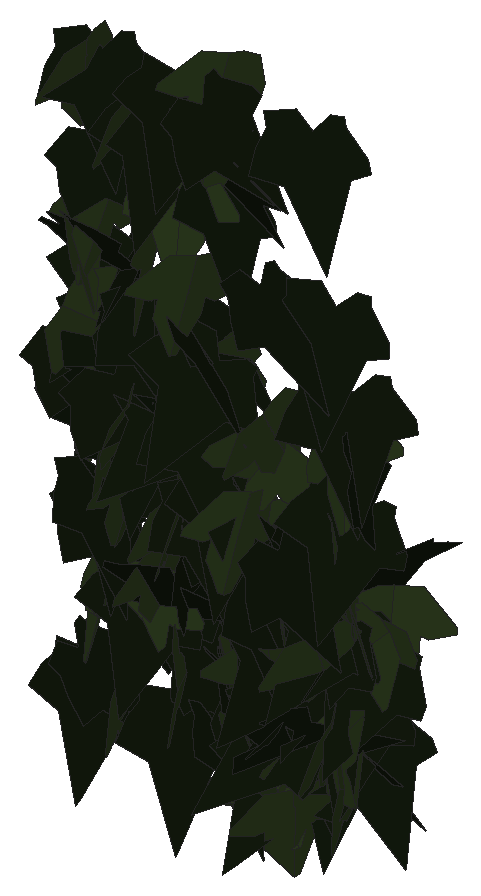
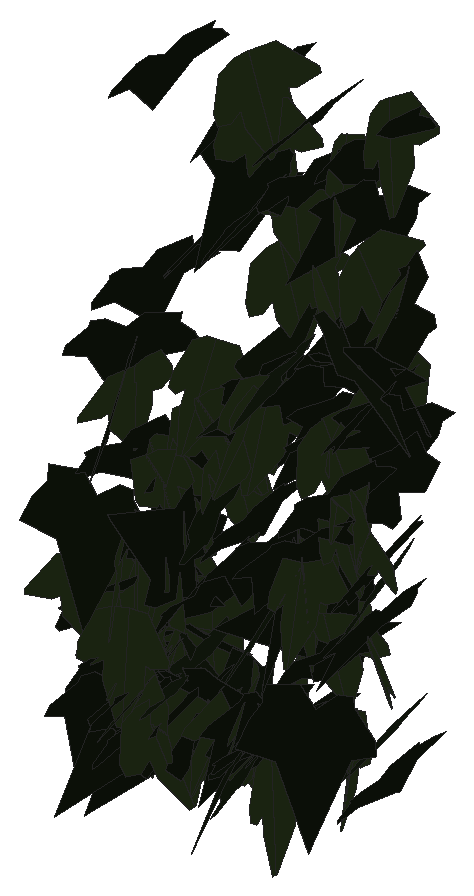
# SketchUp Ruby script. Lengths in inches.
U = 1.inch
M = Sketchup.active_model
def pt(a) = Geom::Point3d.new(a.map { |v| v * U })
def face(e, loops, mat)
  f = e.add_face(loops[0].map { |a| pt(a) })
  loops[1..].each { |l| e.add_face(l.map { |a| pt(a) }).erase! }
  f.material = f.back_material = mat if mat
  f
end
# faces: each face lists its corners as indices into pts; further lists are holes
def faces(e, pts, list, mat = nil) = list.each { |f| face(e, (f[0].is_a?(Array) ? f : [f]).map { |l| l.map { |i| pts[i] } }, mat) }
# xy, xz, yz: faces in a plane at the given z, y or x. An outline is a flat list of corners, or four numbers for a rectangle; further outlines are holes
def ring(l) = l.size == 4 ? [[l[0], l[1]], [l[2], l[1]], [l[2], l[3]], [l[0], l[3]]] : l.each_slice(2).to_a
def flat(e, list, mat, &to3) = list.each { |f| face(e, (f[0].is_a?(Array) ? f : [f]).map { |l| ring(l).map { |u, v| to3.(u, v) } }, mat) }
def xy(e, z, list, mat = nil) = flat(e, list, mat) { |x, y| [x, y, z] }
def xz(e, y, list, mat = nil) = flat(e, list, mat) { |x, z| [x, y, z] }
def yz(e, x, list, mat = nil) = flat(e, list, mat) { |y, z| [x, y, z] }
def lines(e, pts, list) = list.each { |a, b| e.add_line(pt(pts[a]), pt(pts[b])) }
# prism: a flat outline (further loops are holes) pulled along v
def prism(e, loops, v, mat = nil)
  f = face(e, loops, mat); d = Geom::Vector3d.new(v.map { |x| x * U })
  f.pushpull(f.normal.samedirection?(d) ? d.length : -d.length)
end
def box(e, o, s, mat = nil) = prism(e, [[o, [o[0] + s[0], o[1], o[2]], [o[0] + s[0], o[1] + s[1], o[2]], [o[0], o[1] + s[1], o[2]]]], [0, 0, s[2]], mat)
def at(x, y, z, deg = 0) = Geom::Transformation.translation(pt([x, y, z])) * Geom::Transformation.rotation(ORIGIN, Z_AXIS, deg.degrees)
def axes(o, x, y, z) = Geom::Transformation.new([*x, 0, *y, 0, *z, 0, *pt(o).to_a, 1])
def part(name) = M.definitions.add(name)
# library, detail: a bought-in or finely detailed component or shape, given as its bounding box
def library(name, o, s) = part(name).tap { |d| box(d.entities, o, s) }
def detail(e, o, s) = box(e.add_group.entities, o, s)
def put(e, d, t, mat = nil) = e.add_instance(d, t).tap { |i| i.material = mat if mat }
def group(e, t, mat = nil) = e.add_group.tap { |g| g.transformation = t; g.material = mat if mat }.entities
root = M.entities
M.materials.add("efeu1").color = [18, 25, 13]
M.materials.add("efeu2").color = [43, 57, 29]
c1 = part("ivyleaf_9")
p = [[1.54,2.16,1.25],[1.36,2.04,1.19],[-0.21,0.99,0.68],[-0.71,1.11,0.82],[-0.85,0.86,0.67],[-0.8,0.17,0.21],
  [-0.9,-0.01,0.1],[-0.67,-0.16,-0.02],[-0.08,-0.08,-0.05],[-0.03,-0.6,-0.4],[0.65,-0.88,-0.66],[0.83,-0.6,-0.49],
  [1.29,-0.42,-0.43],[1.8125,-0.07,-0.26],[1.21,0.44,0.15]]
faces(c1.entities,p,[[0,1,2,3,4,5,6,7,8,9,10,11,12,13,14]],"efeu1")
c2 = part("ivyleaf_10")
p = [[0,0.5,-0.03],[-0.0625,2.02,-0.43],[-0.19,2.01,-0.46],[-0.54,1.05,-0.29],[-0.52,0.625,-0.18],[-0.83,0.76,-0.28],
  [-1.16,0.64,-0.33],[-1.15,0.33,-0.24],[-0.77,-0.39,0.02],[-0.3,-0.51,0.16],[0.04,-0.48,0.23],[-0.02,2.01,-0.4375],
  [-0.06,2.01,-0.43],[0.04,-0.49,0.23],[0.67,-0.49,0.14],[1.38,0.36,-0.2],[1.375,0.51,-0.24],[0.81,0.65,-0.19],
  [0.62,0.59,-0.15],[0.6,1.09,-0.28],[0.5,1.23,-0.31]]
faces(c2.entities,p,[[0,1,2,3,4,5,6,7,8,9,10],[11,12,0,13,14,15,16,17,18,19,20]],"efeu2")
put(root,c1,axes([30.55,222.95,235.93],[0.19386,-0.41787,-0.19443],[-0.01892,0.20353,-0.45631],[0.4605,0.18427,0.0631]))
put(root,c2,axes([30.73,222.43,239.54],[-0.161,0.47233,-0.03139],[0.01068,-0.02953,-0.49901],[-0.47325,-0.16135,-0.00058]))
put(root,c2,axes([30.82,222.4,241.56],[-0.01451,-0.49272,-0.08377],[0.02037,0.08315,-0.49262],[0.49937,-0.01771,0.01766]))
put(root,c1,axes([30.64,222.81,233.83],[-0.031,-0.48215,0.12872],[0.01205,-0.12966,-0.48275],[0.49889,-0.02683,0.01966]))
put(root,c2,axes([30.57,223.07,236.89],[0.34889,-0.11485,0.33924],[0.31911,-0.11535,-0.36724],[0.16261,0.47276,-0.00719]))
put(root,c1,axes([31.01,222.9,238.78],[-0.45891,-0.19762,-0.01859],[0.01587,0.01014,-0.49965],[0.19786,-0.45918,-0.00303]))
put(root,c1,axes([30.65,222.49,238.12],[0.11578,-0.27785,-0.39924],[0.07613,0.41569,-0.26722],[0.48042,0.00109,0.13856]))
put(root,c1,axes([30.69,222.55,234.3],[0.33786,-0.2932,-0.22335],[-0.07021,0.24625,-0.42946],[0.36183,0.32155,0.12523]))
put(root,c1,axes([30.61,222.39,239.41],[0.48865,-0.03264,0.10078],[0.10352,0.04619,-0.48698],[0.02248,0.49679,0.0519]))
put(root,c1,axes([31.18,222.78,239.02],[-0.34279,0.364,0.00184],[-0.00557,-0.00272,-0.49996],[-0.36396,-0.34278,0.00592]))
put(root,c2,axes([30.81,222.3,238.54],[-0.08236,-0.30647,-0.38639],[0.21642,0.32954,-0.30751],[0.44315,-0.2179,0.07837]))
put(root,c1,axes([30.73,222.92,235.98],[0.09408,-0.44344,0.21097],[0.04085,-0.20699,-0.45331],[0.48937,0.10253,-0.00272]))
put(root,c2,axes([30.97,222.63,239.85],[-0.08362,-0.45117,0.19862],[0.05349,-0.20858,-0.45126],[0.49005,-0.05422,0.08315]))
put(root,c1,axes([31.04,223.44,234.74],[0.279,0.35016,-0.22258],[-0.13361,-0.17811,-0.44769],[-0.39282,0.30929,-0.00582]))
put(root,c1,axes([30.77,222.76,238.31],[0.17898,-0.45059,-0.1222],[-0.01558,0.12504,-0.48386],[0.46661,0.17701,0.03072]))
put(root,c2,axes([30.92,222.64,235.36],[0.36046,-0.31356,0.14749],[0.09884,-0.11095,-0.47741],[0.33212,0.37333,-0.018]))
put(root,c1,axes([30.86,222.68,241.45],[-0.01708,-0.48793,-0.10783],[0.00054,0.10788,-0.48822],[0.49971,-0.01679,-0.00316]))
put(root,c1,axes([30.83,222.6,236.33],[0.14816,-0.47731,-0.01509],[-0.00189,0.01521,-0.49977],[0.47754,0.14815,0.0027]))
put(root,c2,axes([31.15,222.34,237.14],[0.18383,-0.33982,-0.31738],[-0.04232,0.32764,-0.37531],[0.46305,0.16485,0.0917]))
put(root,c2,axes([31.19,222.97,237.81],[-0.168,-0.44111,0.16491],[0.01098,-0.17872,-0.46684],[0.4708,-0.15323,0.06974]))
put(root,c2,axes([31.18,222.54,234.0625],[0.20112,-0.37951,-0.25598],[0.00848,0.28264,-0.41236],[0.45769,0.16152,0.12013]))
put(root,c1,axes([30.98,222.48,240.6],[0.10051,-0.28357,-0.39935],[0.0266,0.41023,-0.28461],[0.48907,0.03597,0.09755]))
put(root,c1,axes([30.8125,222.39,237.12],[0.07192,-0.02937,0.49393],[0.47234,-0.14459,-0.07737],[0.14738,0.47774,0.00695]))
put(root,c1,axes([31.13,223.06,237.22],[-0.09608,-0.49043,-0.01568],[-0.00654,0.01726,-0.49966],[0.49064,-0.09581,-0.00973]))
put(root,c2,axes([31.29,222.5625,241.02],[0.04981,-0.44926,-0.21373],[0.00318,0.21508,-0.45136],[0.4975,0.0436,0.02428]))
put(root,c2,axes([31.35,222.48,237.45],[0.024,-0.39949,-0.29972],[-0.01831,0.29916,-0.40021],[0.49909,0.03019,-0.00026]))
put(root,c2,axes([31.4,222.55,236.73],[0.02853,-0.49666,0.0502],[-0.00165,-0.05037,-0.49745],[0.49918,0.02822,-0.00451]))
put(root,c1,axes([31.38,222.87,235.125],[-0.14875,-0.47153,0.07437],[0.01814,-0.08343,-0.49266],[0.47702,-0.14387,0.04193]))
put(root,c2,axes([31.46,222.64,235.29],[0.47155,0.16207,-0.03714],[-0.03748,-0.00522,-0.49857],[-0.16199,0.47298,0.00722]))
put(root,c2,axes([31.53,223.02,236.11],[-0.06155,-0.46338,-0.17744],[0.05462,0.17139,-0.46652],[0.49318,-0.07682,0.02952]))
put(root,c1,axes([31.3,222.375,237.85],[0.04457,-0.30022,-0.39734],[0.10509,0.39562,-0.28713],[0.4868,-0.05792,0.09836]))
put(root,c1,axes([31.4,222.84,238.54],[0.02355,-0.45825,-0.19863],[0.01148,0.1993,-0.45842],[0.49931,0.01703,0.01991]))
put(root,c2,axes([31.63,223.375,233.73],[0.01446,-0.48813,-0.10733],[0.00744,0.10758,-0.48823],[0.49974,0.01252,0.01038]))
put(root,c1,axes([31.43,223.23,236.5625],[0.03208,-0.45675,-0.20087],[0.05566,0.2033,-0.4534],[0.49586,0.00673,0.06388]))
put(root,c2,axes([31.71,222.61,235.76],[-0.02973,-0.49429,-0.06923],[0.01444,0.06848,-0.49508],[0.49891,-0.03144,0.0102]))
put(root,c1,axes([31.61,222.86,240.84],[-0.18609,-0.46401,0.00784],[0.00313,-0.0097,-0.4999],[0.46407,-0.186,0.00651]))
put(root,c2,axes([31.59,222.62,239.53],[0.19992,-0.39705,0.22888],[0.14752,-0.18067,-0.44226],[0.4339,0.24436,0.04491]))
put(root,c2,axes([31.8,222.7,236.28],[0.21002,-0.40487,-0.20487],[-0.06846,0.19489,-0.45533],[0.44856,0.21931,0.02643]))
put(root,c1,axes([31.92,222.71,235.84],[0.06542,0.0152,-0.49547],[-0.42118,0.26524,-0.04747],[0.2614,0.42357,0.04751]))
put(root,c1,axes([31.41,222.43,235.37],[0.39266,-0.0311,0.30798],[0.30948,0.05005,-0.38951],[-0.0066,0.49652,0.05855]))
put(root,c1,axes([31.625,223.27,235.9],[0.3233,-0.32847,-0.19387],[-0.13214,0.14195,-0.46086],[0.35779,0.34923,0.00498]))
put(root,c1,axes([31.86,222.8125,237.4],[-0.30363,-0.32609,0.22687],[-0.04053,-0.25863,-0.42599],[0.39518,-0.27708,0.13063]))
put(root,c1,axes([31.79,223.6,234.2],[-0.19158,-0.41714,0.19821],[-0.00044,-0.21442,-0.45169],[0.46184,-0.17325,0.08179]))
put(root,c2,axes([32.03,222.99,238.02],[-0.22797,-0.41601,-0.158],[0.06403,0.14501,-0.47421],[0.44038,-0.23644,-0.01284]))
put(root,c2,axes([32.17,222.25,234.56],[0.08439,-0.16014,-0.46608],[-0.14149,0.44509,-0.17855],[0.47208,0.16202,0.02981]))
put(root,c1,axes([31.88,222.71,241.23],[-0.0746,-0.45815,0.18584],[0.04996,-0.19397,-0.45813],[0.49187,-0.04978,0.07471]))
put(root,c1,axes([31.76,223.17,238.46],[0.32641,-0.37095,-0.07649],[0.02465,0.12157,-0.48437],[0.37795,0.31243,0.09765]))
put(root,c1,axes([31.9,223.25,234.46],[0.08686,-0.35585,-0.34033],[-0.05688,0.33602,-0.36586],[0.4891,0.10227,0.01789]))
put(root,c2,axes([31.96,222.58,240.3],[0.47432,0.15581,0.02731],[0.02793,0.00247,-0.49921],[-0.1557,0.4751,-0.00636]))
put(root,c2,axes([32.08,223.13,237.84],[-0.00469,-0.28177,-0.41302],[0.0513,0.41059,-0.28069],[0.49734,-0.04501,0.02506]))
put(root,c1,axes([32.1,223.24,234.14],[0.3005,-0.0699,-0.39347],[-0.33225,0.22985,-0.29458],[0.22206,0.4385,0.09169]))
put(root,c1,axes([31.98,222.61,233.91],[-0.02367,-0.49902,0.02048],[-0.00309,-0.02036,-0.49958],[0.49943,-0.02378,-0.00212]))
put(root,c2,axes([32.2,222.48,239.39],[-0.2023,-0.44647,0.09868],[-0.00346,-0.1064,-0.48853],[0.45723,-0.19835,0.03996]))
put(root,c1,axes([32,223.06,236.31],[-0.00704,-0.48078,-0.13711],[0.04372,0.13601,-0.47916],[0.49804,-0.01873,0.04012]))
put(root,c2,axes([32.18,223.15,234.47],[-0.25616,0.42938,0.00423],[0.00285,0.00662,-0.49995],[-0.42939,-0.25611,-0.00584]))
put(root,c1,axes([32.24,222.82,238.16],[-0.29321,-0.39613,0.08433],[-0.02372,-0.08713,-0.49178],[0.40431,-0.29239,0.0323]))
put(root,c2,axes([32.4,222.62,241.1],[-0.46392,-0.13327,0.13044],[-0.11669,-0.06533,-0.48178],[0.14546,-0.47746,0.02951]))
put(root,c1,axes([31.97,222.76,238.48],[0.27347,-0.37916,0.17735],[0.10254,-0.1447,-0.46749],[0.40583,0.29206,-0.00139]))
put(root,c2,axes([32.4,222.76,241.75],[-0.2242,-0.43112,0.11778],[0.00432,-0.13386,-0.48173],[0.4469,-0.21499,0.06375]))
put(root,c1,axes([32.17,223.07,233.63],[0.2215,-0.43994,0.08599],[0.03415,-0.07908,-0.49252],[0.44696,0.22406,-0.00498]))
put(root,c1,axes([32.3,223.04,236.5],[-0.04344,-0.48481,0.11435],[0.01277,-0.11583,-0.48623],[0.49795,-0.03933,0.02244]))
put(root,c1,axes([32.3,222.96,240.19],[0.06933,-0.49443,0.02704],[0.00082,-0.02719,-0.49926],[0.49517,0.06928,-0.00296]))
put(root,c1,axes([32.35,222.62,237.63],[-0.13283,-0.44527,-0.18464],[0.08351,0.16737,-0.4637],[0.47474,-0.15403,0.0299]))
put(root,c2,axes([32.47,223.17,234.19],[-0.07953,0.45786,0.18449],[-0.03143,0.18179,-0.46472],[-0.49263,-0.08552,-0.00013]))
put(root,c1,axes([32.41,222.62,240.72],[0.4719,0.06564,-0.15165],[-0.15406,0.00879,-0.47559],[-0.05977,0.4956,0.02852]))
put(root,c1,axes([32.16,223.21,234.23],[0.38781,-0.2491,0.19379],[0.18308,-0.07252,-0.45959],[0.25707,0.42743,0.03496]))
put(root,c1,axes([32.76,223.34,234.47],[-0.49295,-0.08366,0.00105],[-0.0005,-0.00333,-0.49999],[0.08366,-0.49294,0.0032]))
put(root,c1,axes([32.55,222.28,241.56],[0.21033,-0.32397,-0.3175],[-0.07118,0.32206,-0.37578],[0.44799,0.20328,0.08936]))
put(root,c2,axes([33.07,222.41,233.84],[-0.35172,0.07379,0.34764],[-0.34624,0.03906,-0.3586],[-0.08008,-0.49298,0.02362]))
put(root,c1,axes([32.51,223.23,236.625],[0.20902,-0.38984,0.2331],[0.10476,-0.20831,-0.4423],[0.44197,0.23375,-0.0054]))
put(root,c2,axes([32.86,222.51,236.76],[-0.14145,-0.46214,0.12813],[0.0464,-0.14614,-0.47591],[0.47733,-0.12274,0.08423]))
put(root,c2,axes([33.02,222.71,237.37],[0.37092,0.21435,-0.25782],[-0.28743,0.00531,-0.40909],[-0.17264,0.45169,0.12716]))
put(root,c1,axes([32.8,223.24,235.49],[-0.13421,-0.45946,0.1445],[-0.00728,-0.14806,-0.47752],[0.4816,-0.13028,0.03305]))
put(root,c2,axes([33.04,223.56,234.01],[-0.25408,-0.39671,0.16754],[-0.09353,-0.13904,-0.47108],[0.42035,-0.27072,-0.00355]))
put(root,c1,axes([32.83,223.07,234.23],[0.15701,-0.43232,-0.19607],[-0.04361,0.1925,-0.45939],[0.4727,0.16136,0.02275]))
put(root,c2,axes([32.75,222.92,233.66],[0.37036,0.109,0.31773],[0.29362,0.12466,-0.38503],[-0.16315,0.47178,0.02833]))
put(root,c2,axes([33.15,222.58,235.01],[-0.37931,-0.32345,0.0388],[-0.03371,-0.02026,-0.49845],[0.32401,-0.38075,-0.00644]))
put(root,c1,axes([32.79,223.36,234.65],[0.18404,-0.45409,0.09967],[0.1051,-0.06378,-0.48465],[0.45286,0.19934,0.07198]))
put(root,c1,axes([32.91,222.9,235.49],[0.11888,-0.48544,0.01465],[0.00306,-0.01433,-0.49979],[0.48565,0.11892,-0.00043]))
put(root,c1,axes([33.04,223.04,235.78],[0.01388,-0.06907,0.49501],[0.3203,0.38138,0.04424],[-0.38369,0.31587,0.05483]))
put(root,c2,axes([33.15,222.56,237.89],[-0.11456,-0.42071,-0.2447],[0.08403,0.23051,-0.43566],[0.47939,-0.14094,0.01789]))
put(root,c1,axes([33.31,222.86,233.85],[-0.35476,-0.35042,0.0368],[-0.02316,-0.02892,-0.49863],[0.35158,-0.35549,0.00429]))
put(root,c1,axes([33.25,222.81,235.04],[-0.1697,-0.37948,0.27784],[-0.08191,-0.26701,-0.41472],[0.46313,-0.18627,0.02845]))
put(root,c2,axes([33.23,222.87,235.11],[-0.24317,0.43639,-0.0208],[0.02145,-0.01185,-0.4994],[-0.43636,-0.24377,-0.01296]))
put(root,c1,axes([33.51,222.6,234.38],[-0.48519,-0.10072,0.06665],[-0.06366,-0.02117,-0.49548],[0.10263,-0.48929,0.00772]))
put(root,c1,axes([33.56,222.375,234.68],[-0.12621,0.42572,0.22986],[-0.11169,0.2055,-0.44192],[-0.47074,-0.16289,0.04323]))
put(root,c1,axes([33.14,223.28,233.97],[0.49427,0.0528,-0.05398],[-0.05434,0.00048,-0.49704],[-0.05243,0.4972,0.00621]))
put(root,c2,axes([33.37,223.2,235.44],[-0.47472,0.15695,-0.00342],[-0.00081,-0.01335,-0.49982],[-0.15698,-0.47454,0.01293]))
put(root,c2,axes([33.52,222.92,236.58],[0.41609,-0.04143,-0.27414],[-0.26804,0.06627,-0.41685],[0.07088,0.49385,0.03294]))
put(root,c2,axes([33.1875,222.58,233.93],[0.38786,0.27104,0.16156],[0.13442,0.08968,-0.47317],[-0.28548,0.41048,-0.0033]))
put(root,c1,axes([33.16,222.47,239.52],[0.24045,-0.41654,-0.13667],[-0.01117,0.15,-0.47684],[0.43824,0.23237,0.06283]))
put(root,c2,axes([33.52,223.58,234.9375],[-0.49074,0.01591,0.09446],[-0.09453,-0.00081,-0.49098],[-0.01547,-0.49975,0.00381]))
put(root,c2,axes([33.03,223.61,234],[0.02724,0.00534,0.49923],[0.49689,-0.04895,-0.02659],[0.04859,0.49757,-0.00797]))
put(root,c2,axes([33.47,222.89,233.85],[0.00782,-0.44792,0.22206],[0.01362,-0.22181,-0.4479],[0.49975,0.01305,0.00873]))
put(root,c1,axes([33.31,223.4,234.16],[-0.09987,-0.4758,-0.11678],[0.03326,0.11233,-0.48608],[0.48879,-0.10486,0.00922]))
put(root,c1,axes([33.19,223.64,234.4375],[0.20733,-0.4545,0.02111],[0.0202,-0.01398,-0.4994],[0.45454,0.20793,0.01257]))
put(root,c2,axes([33.375,222.7,234.47],[0.4603,0.19499,-0.01033],[-0.0096,-0.00382,-0.49989],[-0.19503,0.4604,0.00022]))
put(root,c2,axes([33.62,222.83,236.67],[0.35584,-0.18705,-0.29731],[-0.20495,0.23313,-0.39198],[0.28526,0.40083,0.08924]))
put(root,c1,axes([33.38,223.45,233.81],[-0.05543,-0.49546,0.038],[-0.00019,-0.03822,-0.49854],[0.49692,-0.05528,0.00405]))
put(root,c2,axes([33.59,222.44,233.56],[-0.24384,-0.43507,-0.03546],[0.01365,0.033,-0.49872],[0.4363,-0.24419,-0.00421]))
put(root,c2,axes([33.53,223.08,234.42],[-0.04639,0.49695,0.0298],[-0.02294,0.02776,-0.4987],[-0.49731,-0.04764,0.02023]))
put(root,c2,axes([33.53,223.21,235.86],[0.42393,-0.25451,-0.07424],[0.0322,0.18842,-0.46202],[0.26315,0.38694,0.17614]))
put(root,c1,axes([33.66,223.01,235.38],[-0.42819,-0.2119,-0.14748],[0.13056,0.06868,-0.47774],[0.22272,-0.44764,-0.00349]))
put(root,c1,axes([33.375,222.23,234.26],[0.08667,0.2718,-0.41062],[0.14183,0.38549,0.2851],[0.47156,-0.16589,-0.01027]))
put(root,c1,axes([33.59,223.12,239.13],[-0.10959,-0.4847,-0.05526],[0.00032,0.05657,-0.49679],[0.48784,-0.10892,-0.01209]))
put(root,c1,axes([33.55,222.29,236.57],[0.16644,-0.36529,-0.2981],[-0.11917,0.27327,-0.4014],[0.45617,0.20467,0.0039]))
put(root,c1,axes([33.75,223.16,235.55],[-0.34044,-0.3512,0.10372],[-0.02686,-0.11729,-0.48531],[0.36521,-0.33601,0.061]))
put(root,c1,axes([33.53,223.31,233.85],[0.49196,0.02107,-0.08676],[-0.08812,0.03626,-0.49084],[-0.01439,0.49824,0.03939]))
put(root,c2,axes([33.91,223.28,235.38],[-0.44988,-0.1544,0.15419],[-0.14381,-0.05593,-0.4756],[0.16411,-0.47226,0.00592]))
put(root,c2,axes([33.79,222.58,235.41],[-0.22707,-0.42312,-0.13933],[0.06888,0.12116,-0.48018],[0.44011,-0.23726,0.00327]))
put(root,c2,axes([33.93,223.09,235.63],[-0.26812,0.30781,0.28873],[-0.20902,0.20032,-0.40766],[-0.36664,-0.3393,0.02125]))
put(root,c1,axes([33.74,223.42,234.51],[-0.15211,-0.47626,0.00619],[0.00915,-0.00942,-0.49983],[0.47621,-0.15195,0.01158]))
put(root,c2,axes([33.78,223.11,233.86],[0.40671,-0.28798,0.04067],[0.0347,-0.02138,-0.49834],[0.28876,0.40818,0.0026]))
put(root,c2,axes([33.88,222.67,234.4],[0.10334,-0.43877,-0.21633],[-0.00961,0.21924,-0.44927],[0.48911,0.09701,0.03688]))
put(root,c2,axes([33.78,223.09,237.7],[0.13067,0.47683,-0.07455],[-0.02734,-0.0698,-0.49435],[-0.48185,0.13327,0.00783]))
put(root,c2,axes([34.07,223.13,235.36],[0.36344,-0.09126,-0.33103],[-0.31528,0.10228,-0.37435],[0.13604,0.48084,0.0168]))
put(root,c1,axes([33.7,222.63,241.47],[-0.00049,-0.49417,-0.07612],[0.01775,0.07605,-0.49386],[0.49968,-0.00319,0.01747]))
put(root,c1,axes([34.11,222.79,237.54],[0.12403,0.12539,-0.46786],[-0.43698,0.23731,-0.05224],[0.20896,0.42185,0.16845]))
put(root,c1,axes([34.11,223.3125,236.21],[0.12146,0.48501,0.00364],[-0.08016,0.02377,-0.49296],[-0.47835,0.11917,0.08354]))
put(root,c1,axes([33.92,223.07,236.86],[-0.19131,-0.46153,0.01983],[0.00811,-0.02481,-0.49932],[0.46188,-0.19072,0.01698]))
put(root,c2,axes([34.08,222.6,233.85],[0.12624,-0.23932,-0.42046],[-0.06924,0.42113,-0.26049],[0.47882,0.12399,0.07319]))
put(root,c1,axes([33.9,223.04,238.24],[-0.19127,-0.41248,-0.20802],[0.08234,0.1911,-0.45464],[0.45457,-0.20818,-0.00517]))
put(root,c2,axes([33.74,222.85,234.04],[0.28653,-0.23234,-0.33751],[0.26389,-0.21043,0.36889],[-0.31347,-0.38953,0.00204]))
put(root,c2,axes([34,223.56,235.53],[0.34871,0.35755,-0.0236],[-0.06831,0.03401,-0.49414],[-0.35176,0.34785,0.07257]))
put(root,c1,axes([34.02,223.34,235.05],[-0.26593,-0.42009,0.05292],[0.00754,-0.06718,-0.49541],[0.42335,-0.26269,0.04207]))
put(root,c1,axes([33.89,223.34,234.09],[-0.03268,-0.42895,-0.25482],[0.0119,0.25462,-0.43015],[0.49879,-0.03418,-0.00643]))
